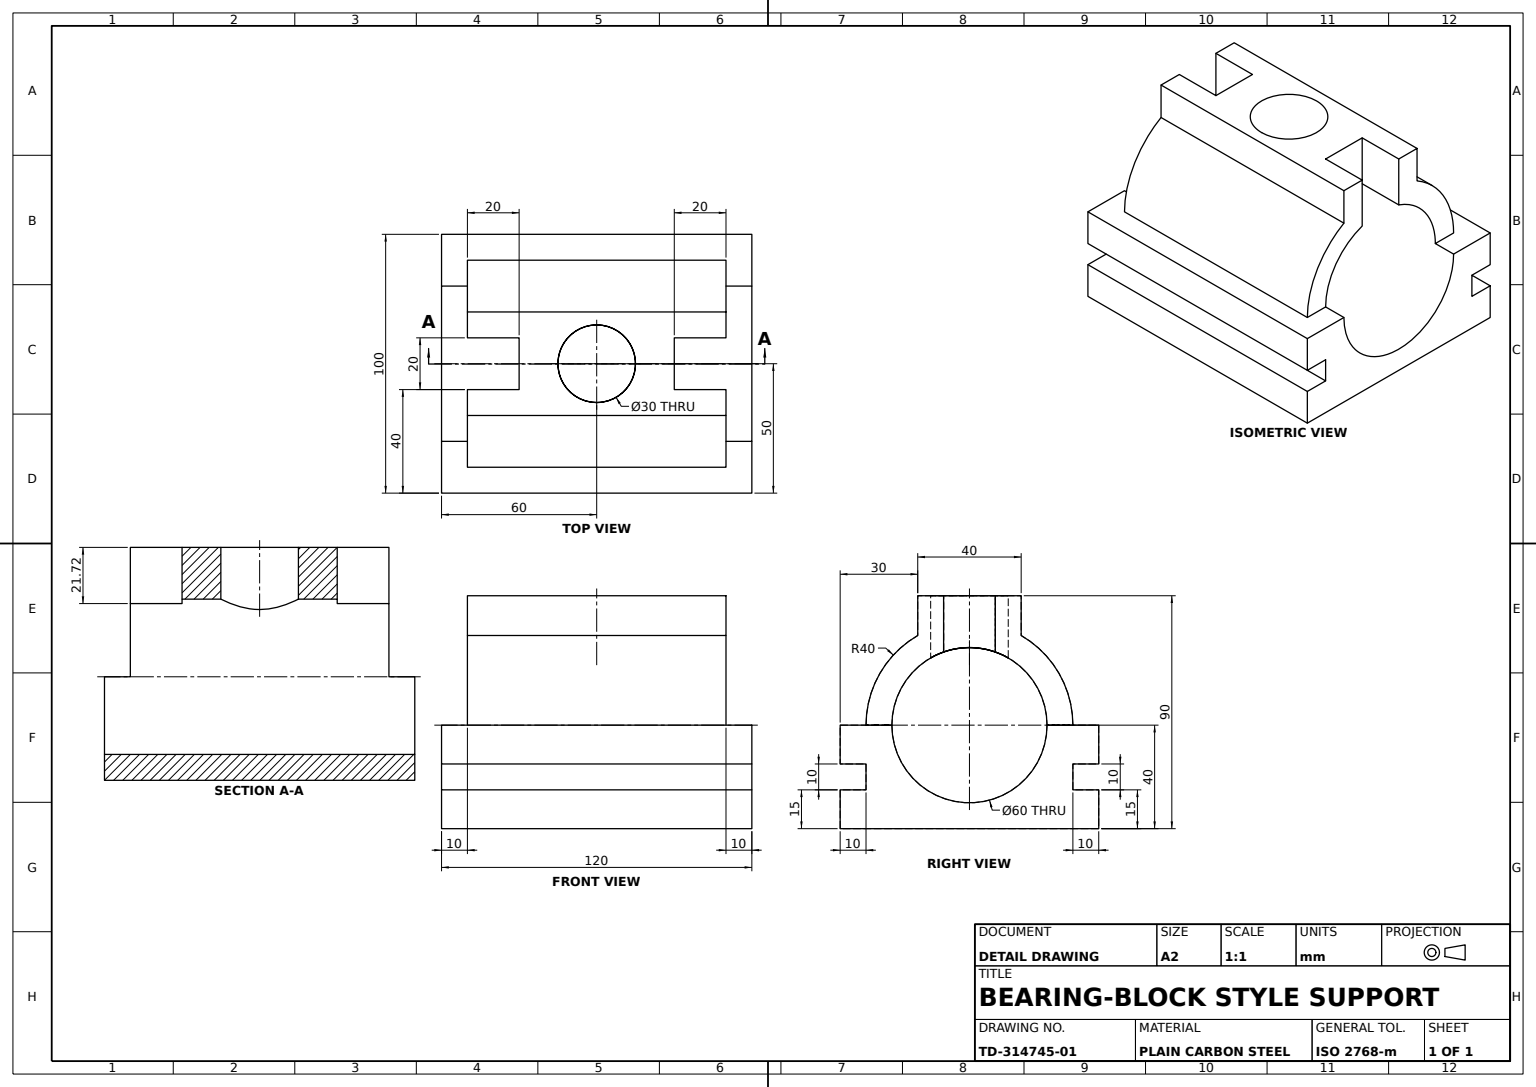
ISO-10303-21;
HEADER;
FILE_DESCRIPTION((''),'2;1');
FILE_NAME('','',(''),(''),'','','');
FILE_SCHEMA(('AUTOMOTIVE_DESIGN'));
ENDSEC;
DATA;
#1=APPLICATION_CONTEXT('');
#2=PRODUCT_CONTEXT('',#1,'mechanical');
#3=PRODUCT('','','',(#2));
#4=PRODUCT_DEFINITION_FORMATION('','',#3);
#5=PRODUCT_DEFINITION_CONTEXT('',#1,'design');
#6=PRODUCT_DEFINITION('','',#4,#5);
#7=PRODUCT_DEFINITION_SHAPE('','',#6);
#8=(LENGTH_UNIT()NAMED_UNIT(*)SI_UNIT(.MILLI.,.METRE.));
#9=(NAMED_UNIT(*)PLANE_ANGLE_UNIT()SI_UNIT($,.RADIAN.));
#10=(NAMED_UNIT(*)SI_UNIT($,.STERADIAN.)SOLID_ANGLE_UNIT());
#11=UNCERTAINTY_MEASURE_WITH_UNIT(LENGTH_MEASURE(1.E-05),#8,'distance_accuracy_value','');
#12=(GEOMETRIC_REPRESENTATION_CONTEXT(3)GLOBAL_UNCERTAINTY_ASSIGNED_CONTEXT((#11))GLOBAL_UNIT_ASSIGNED_CONTEXT((#8,#9,#10))REPRESENTATION_CONTEXT('',''));
#13=CARTESIAN_POINT('',(65.,65.980762,-60.));
#14=VERTEX_POINT('',#13);
#15=CARTESIAN_POINT('',(35.,65.980762,-60.));
#16=VERTEX_POINT('',#15);
#17=CARTESIAN_POINT('',(65.,65.980762,-59.503514));
#18=CARTESIAN_POINT('',(64.975416,65.995004,-59.005113));
#19=CARTESIAN_POINT('',(64.875156,66.052506,-58.004351));
#20=CARTESIAN_POINT('',(64.800107,66.095393,-57.509543));
#21=CARTESIAN_POINT('',(64.505151,66.261216,-56.052494));
#22=CARTESIAN_POINT('',(64.215664,66.421584,-55.11219));
#23=CARTESIAN_POINT('',(63.451904,66.818491,-53.290153));
#24=CARTESIAN_POINT('',(62.989124,67.048728,-52.435825));
#25=CARTESIAN_POINT('',(62.180532,67.417556,-51.232551));
#26=CARTESIAN_POINT('',(61.891675,67.544511,-50.844443));
#27=CARTESIAN_POINT('',(61.274128,67.802987,-50.093931));
#28=CARTESIAN_POINT('',(60.947936,67.933407,-49.734782));
#29=CARTESIAN_POINT('',(59.926264,68.319595,-48.712961));
#30=CARTESIAN_POINT('',(59.184727,68.571758,-48.101049));
#31=CARTESIAN_POINT('',(57.975732,68.923413,-47.286867));
#32=CARTESIAN_POINT('',(57.553955,69.036776,-47.03168));
#33=CARTESIAN_POINT('',(56.69248,69.247347,-46.566822));
#34=CARTESIAN_POINT('',(56.252173,69.344857,-46.356378));
#35=CARTESIAN_POINT('',(54.902311,69.610955,-45.790156));
#36=CARTESIAN_POINT('',(53.964123,69.753262,-45.498737));
#37=CARTESIAN_POINT('',(52.49344,69.900259,-45.200237));
#38=CARTESIAN_POINT('',(51.995929,69.937639,-45.125052));
#39=CARTESIAN_POINT('',(51.005292,69.987253,-45.025448));
#40=CARTESIAN_POINT('',(50.50939,69.999784,-45.000433));
#41=CARTESIAN_POINT('',(49.516426,70.000211,-44.999578));
#42=CARTESIAN_POINT('',(49.019365,69.988108,-45.023737));
#43=CARTESIAN_POINT('',(48.024058,69.939003,-45.122307));
#44=CARTESIAN_POINT('',(47.524118,69.901685,-45.197361));
#45=CARTESIAN_POINT('',(46.059254,69.756237,-45.492658));
#46=CARTESIAN_POINT('',(45.117292,69.614488,-45.78273));
#47=CARTESIAN_POINT('',(43.753408,69.34612,-46.353645));
#48=CARTESIAN_POINT('',(43.30559,69.246907,-46.56778));
#49=CARTESIAN_POINT('',(42.444004,69.036246,-47.032865));
#50=CARTESIAN_POINT('',(42.028081,68.924446,-47.284536));
#51=CARTESIAN_POINT('',(41.224502,68.690865,-47.825224));
#52=CARTESIAN_POINT('',(40.836849,68.569076,-48.114244));
#53=CARTESIAN_POINT('',(40.089257,68.318415,-48.730053));
#54=CARTESIAN_POINT('',(39.727696,68.188892,-49.058595));
#55=CARTESIAN_POINT('',(38.701032,67.800518,-50.086794));
#56=CARTESIAN_POINT('',(38.091001,67.541355,-50.82898));
#57=CARTESIAN_POINT('',(37.283022,67.172892,-52.030594));
#58=CARTESIAN_POINT('',(37.031694,67.053469,-52.445978));
#59=CARTESIAN_POINT('',(36.566237,66.825383,-53.308645));
#60=CARTESIAN_POINT('',(36.354634,66.717956,-53.751628));
#61=CARTESIAN_POINT('',(35.788686,66.423841,-55.101913));
#62=CARTESIAN_POINT('',(35.499327,66.2637,-56.036017));
#63=CARTESIAN_POINT('',(35.202669,66.09697,-57.493076));
#64=CARTESIAN_POINT('',(35.126663,66.053546,-57.990752));
#65=CARTESIAN_POINT('',(35.025442,65.9955,-58.9921));
#66=CARTESIAN_POINT('',(35.,65.980762,-59.495938));
#67=B_SPLINE_CURVE_WITH_KNOTS('',3,(#13,#17,#18,#19,#20,#21,#22,#23,#24,#25,#26,#27,#28,#29,#30,#31,#32,#33,#34,#35,#36,#37,#38,#39,#40,#41,#42,#43,#44,#45,#46,#47,#48,#49,#50,#51,#52,#53,#54,#55,#56,#57,#58,#59,#60,#61,#62,#63,#64,#65,#66,#15),.UNSPECIFIED.,.F.,.F.,(4,2,2,2,2,2,2,2,2,2,2,2,2,2,2,2,2,2,2,2,2,2,2,2,2,4),(0.047708954,0.049197223,0.050685492,0.053662031,0.05663857,0.058126839,0.059615109,0.062591647,0.064079917,0.065568186,0.068544725,0.070032994,0.071521263,0.073009533,0.074497802,0.077474341,0.07896261,0.08045088,0.081939149,0.083427418,0.086403957,0.087892226,0.089380496,0.092357035,0.093845304,0.095333573),.UNSPECIFIED.);
#68=EDGE_CURVE('',#14,#16,#67,.T.);
#69=ORIENTED_EDGE('',*,*,#68,.F.);
#70=CARTESIAN_POINT('',(35.,65.980762,-61.00991));
#71=CARTESIAN_POINT('',(35.100904,66.039726,-61.998787));
#72=CARTESIAN_POINT('',(35.394482,66.204798,-63.453028));
#73=CARTESIAN_POINT('',(35.516241,66.272578,-63.932899));
#74=CARTESIAN_POINT('',(35.808323,66.431496,-64.88296));
#75=CARTESIAN_POINT('',(35.977469,66.521955,-65.348671));
#76=CARTESIAN_POINT('',(36.545369,66.817065,-66.703103));
#77=CARTESIAN_POINT('',(37.006104,67.046531,-67.556891));
#78=CARTESIAN_POINT('',(37.820536,67.418054,-68.76913));
#79=CARTESIAN_POINT('',(38.11221,67.546163,-69.160437));
#80=CARTESIAN_POINT('',(38.725978,67.803005,-69.906038));
#81=CARTESIAN_POINT('',(39.049317,67.932321,-70.262249));
#82=CARTESIAN_POINT('',(39.729091,68.189368,-70.942561));
#83=CARTESIAN_POINT('',(40.085524,68.317106,-71.266661));
#84=CARTESIAN_POINT('',(40.832809,68.567778,-71.882638));
#85=CARTESIAN_POINT('',(41.225935,68.691341,-72.175924));
#86=CARTESIAN_POINT('',(42.438815,69.043717,-72.991454));
#87=CARTESIAN_POINT('',(43.292713,69.255022,-73.45243));
#88=CARTESIAN_POINT('',(44.644725,69.521721,-74.019983));
#89=CARTESIAN_POINT('',(45.107337,69.602244,-74.18835));
#90=CARTESIAN_POINT('',(46.058083,69.743777,-74.481324));
#91=CARTESIAN_POINT('',(46.544404,69.804329,-74.604976));
#92=CARTESIAN_POINT('',(48.004312,69.949522,-74.899769));
#93=CARTESIAN_POINT('',(48.990566,69.999671,-74.999343));
#94=CARTESIAN_POINT('',(50.489993,70.000162,-75.000324));
#95=CARTESIAN_POINT('',(50.996371,69.987604,-74.975255));
#96=CARTESIAN_POINT('',(51.993415,69.93786,-74.875393));
#97=CARTESIAN_POINT('',(52.485426,69.900852,-74.800954));
#98=CARTESIAN_POINT('',(53.456927,69.80416,-74.604631));
#99=CARTESIAN_POINT('',(53.936417,69.744472,-74.482743));
#100=CARTESIAN_POINT('',(54.883034,69.6038,-74.191589));
#101=CARTESIAN_POINT('',(55.352688,69.522267,-74.021153));
#102=CARTESIAN_POINT('',(56.719013,69.252639,-73.447338));
#103=CARTESIAN_POINT('',(57.575449,69.039935,-72.982988));
#104=CARTESIAN_POINT('',(58.784985,68.687983,-72.168007));
#105=CARTESIAN_POINT('',(59.177289,68.564556,-71.874929));
#106=CARTESIAN_POINT('',(59.927306,68.312631,-71.25545));
#107=CARTESIAN_POINT('',(60.284308,68.184483,-70.929994));
#108=CARTESIAN_POINT('',(61.303858,67.7984,-69.90706));
#109=CARTESIAN_POINT('',(61.915532,67.538642,-69.163617));
#110=CARTESIAN_POINT('',(62.730469,67.166603,-67.948151));
#111=CARTESIAN_POINT('',(62.982388,67.046685,-67.529497));
#112=CARTESIAN_POINT('',(63.442131,66.821161,-66.674193));
#113=CARTESIAN_POINT('',(63.650903,66.715119,-66.236145));
#114=CARTESIAN_POINT('',(64.026289,66.519954,-65.338527));
#115=CARTESIAN_POINT('',(64.192907,66.430826,-64.878958));
#116=CARTESIAN_POINT('',(64.41013,66.312639,-64.172394));
#117=CARTESIAN_POINT('',(64.477074,66.27583,-63.933999));
#118=CARTESIAN_POINT('',(64.599699,66.207894,-63.451206));
#119=CARTESIAN_POINT('',(64.655474,66.176713,-63.206163));
#120=CARTESIAN_POINT('',(64.902037,66.038059,-61.981814));
#121=CARTESIAN_POINT('',(65.,65.980762,-60.994731));
#122=B_SPLINE_CURVE_WITH_KNOTS('',3,(#15,#70,#71,#72,#73,#74,#75,#76,#77,#78,#79,#80,#81,#82,#83,#84,#85,#86,#87,#88,#89,#90,#91,#92,#93,#94,#95,#96,#97,#98,#99,#100,#101,#102,#103,#104,#105,#106,#107,#108,#109,#110,#111,#112,#113,#114,#115,#116,#117,#118,#119,#120,#121,#13),.UNSPECIFIED.,.F.,.F.,(4,2,2,2,2,2,2,2,2,2,2,2,2,2,2,2,2,2,2,2,2,2,2,2,2,2,4),(0.,0.00298181,0.004472714,0.005963619,0.008945429,0.010436334,0.011927238,0.013418143,0.014909048,0.017890858,0.019381762,0.020872667,0.023854477,0.025345382,0.026836286,0.028327191,0.029818096,0.032799906,0.03429081,0.035781715,0.038763525,0.04025443,0.041745334,0.043236239,0.043981692,0.044727144,0.047708954),.UNSPECIFIED.);
#123=EDGE_CURVE('',#16,#14,#122,.T.);
#124=ORIENTED_EDGE('',*,*,#123,.F.);
#125=EDGE_LOOP('',(#69,#124));
#126=FACE_BOUND('',#125,.T.);
#127=CARTESIAN_POINT('',(40.,68.284271,-10.));
#128=VERTEX_POINT('',#127);
#129=CARTESIAN_POINT('',(40.,68.284271,-30.));
#130=VERTEX_POINT('',#129);
#131=CARTESIAN_POINT('',(40.,68.284271,-120.));
#132=DIRECTION('',(0.,0.,-1.));
#133=VECTOR('',#132,1000.);
#134=LINE('',#131,#133);
#135=EDGE_CURVE('',#128,#130,#134,.T.);
#136=ORIENTED_EDGE('',*,*,#135,.F.);
#137=CARTESIAN_POINT('',(20.,40.,-10.));
#138=VERTEX_POINT('',#137);
#139=CARTESIAN_POINT('',(50.,40.,-10.));
#140=DIRECTION('',(0.,0.,1.));
#141=DIRECTION('',(1.,0.,0.));
#142=AXIS2_PLACEMENT_3D('',#139,#140,#141);
#143=CIRCLE('',#142,30.);
#144=EDGE_CURVE('',#128,#138,#143,.T.);
#145=ORIENTED_EDGE('',*,*,#144,.T.);
#146=CARTESIAN_POINT('',(20.,40.,-110.));
#147=VERTEX_POINT('',#146);
#148=CARTESIAN_POINT('',(20.,40.,-120.));
#149=VECTOR('',#140,1000.);
#150=LINE('',#148,#149);
#151=EDGE_CURVE('',#147,#138,#150,.T.);
#152=ORIENTED_EDGE('',*,*,#151,.F.);
#153=CARTESIAN_POINT('',(40.,68.284271,-110.));
#154=VERTEX_POINT('',#153);
#155=CARTESIAN_POINT('',(50.,40.,-110.));
#156=AXIS2_PLACEMENT_3D('',#155,#140,#141);
#157=CIRCLE('',#156,30.);
#158=EDGE_CURVE('',#154,#147,#157,.T.);
#159=ORIENTED_EDGE('',*,*,#158,.F.);
#160=CARTESIAN_POINT('',(40.,68.284271,-90.));
#161=VERTEX_POINT('',#160);
#162=EDGE_CURVE('',#161,#154,#134,.T.);
#163=ORIENTED_EDGE('',*,*,#162,.F.);
#164=CARTESIAN_POINT('',(60.,68.284271,-90.));
#165=VERTEX_POINT('',#164);
#166=CARTESIAN_POINT('',(50.,40.,-90.));
#167=AXIS2_PLACEMENT_3D('',#166,#140,#141);
#168=CIRCLE('',#167,30.);
#169=EDGE_CURVE('',#165,#161,#168,.T.);
#170=ORIENTED_EDGE('',*,*,#169,.F.);
#171=CARTESIAN_POINT('',(60.,68.284271,-110.));
#172=VERTEX_POINT('',#171);
#173=CARTESIAN_POINT('',(60.,68.284271,-120.));
#174=LINE('',#173,#149);
#175=EDGE_CURVE('',#172,#165,#174,.T.);
#176=ORIENTED_EDGE('',*,*,#175,.F.);
#177=CARTESIAN_POINT('',(80.,40.,-110.));
#178=VERTEX_POINT('',#177);
#179=EDGE_CURVE('',#178,#172,#157,.T.);
#180=ORIENTED_EDGE('',*,*,#179,.F.);
#181=CARTESIAN_POINT('',(80.,40.,-10.));
#182=VERTEX_POINT('',#181);
#183=CARTESIAN_POINT('',(80.,40.,-120.));
#184=LINE('',#183,#149);
#185=EDGE_CURVE('',#178,#182,#184,.T.);
#186=ORIENTED_EDGE('',*,*,#185,.T.);
#187=CARTESIAN_POINT('',(60.,68.284271,-10.));
#188=VERTEX_POINT('',#187);
#189=EDGE_CURVE('',#182,#188,#143,.T.);
#190=ORIENTED_EDGE('',*,*,#189,.T.);
#191=CARTESIAN_POINT('',(60.,68.284271,-30.));
#192=VERTEX_POINT('',#191);
#193=EDGE_CURVE('',#192,#188,#174,.T.);
#194=ORIENTED_EDGE('',*,*,#193,.F.);
#195=CARTESIAN_POINT('',(50.,40.,-30.));
#196=DIRECTION('',(-1.,0.,0.));
#197=AXIS2_PLACEMENT_3D('',#195,#132,#196);
#198=CIRCLE('',#197,30.);
#199=EDGE_CURVE('',#130,#192,#198,.T.);
#200=ORIENTED_EDGE('',*,*,#199,.F.);
#201=EDGE_LOOP('',(#136,#145,#152,#159,#163,#170,#176,#180,#186,#190,#194,#200));
#202=FACE_OUTER_BOUND('',#201,.T.);
#203=CARTESIAN_POINT('',(50.,40.,-120.));
#204=AXIS2_PLACEMENT_3D('',#203,#140,#141);
#205=CYLINDRICAL_SURFACE('',#204,30.);
#206=ADVANCED_FACE('',(#126,#202),#205,.F.);
#207=CARTESIAN_POINT('',(80.,40.,0.));
#208=VERTEX_POINT('',#207);
#209=EDGE_CURVE('',#182,#208,#184,.T.);
#210=ORIENTED_EDGE('',*,*,#209,.T.);
#211=CARTESIAN_POINT('',(100.,40.,0.));
#212=VERTEX_POINT('',#211);
#213=VECTOR('',#196,1000.);
#214=LINE('',#211,#213);
#215=EDGE_CURVE('',#212,#208,#214,.T.);
#216=ORIENTED_EDGE('',*,*,#215,.F.);
#217=CARTESIAN_POINT('',(100.,40.,-120.));
#218=VERTEX_POINT('',#217);
#219=LINE('',#217,#149);
#220=EDGE_CURVE('',#218,#212,#219,.T.);
#221=ORIENTED_EDGE('',*,*,#220,.F.);
#222=VERTEX_POINT('',#183);
#223=LINE('',#217,#213);
#224=EDGE_CURVE('',#218,#222,#223,.T.);
#225=ORIENTED_EDGE('',*,*,#224,.T.);
#226=EDGE_CURVE('',#222,#178,#184,.T.);
#227=ORIENTED_EDGE('',*,*,#226,.T.);
#228=CARTESIAN_POINT('',(90.,40.,-110.));
#229=VERTEX_POINT('',#228);
#230=CARTESIAN_POINT('',(0.,40.,-110.));
#231=VECTOR('',#141,1000.);
#232=LINE('',#230,#231);
#233=EDGE_CURVE('',#178,#229,#232,.T.);
#234=ORIENTED_EDGE('',*,*,#233,.T.);
#235=CARTESIAN_POINT('',(90.,40.,-10.));
#236=VERTEX_POINT('',#235);
#237=LINE('',#228,#149);
#238=EDGE_CURVE('',#229,#236,#237,.T.);
#239=ORIENTED_EDGE('',*,*,#238,.T.);
#240=CARTESIAN_POINT('',(0.,40.,-10.));
#241=LINE('',#240,#231);
#242=EDGE_CURVE('',#182,#236,#241,.T.);
#243=ORIENTED_EDGE('',*,*,#242,.F.);
#244=EDGE_LOOP('',(#210,#216,#221,#225,#227,#234,#239,#243));
#245=FACE_OUTER_BOUND('',#244,.T.);
#246=DIRECTION('',(0.,1.,0.));
#247=AXIS2_PLACEMENT_3D('',#217,#246,#140);
#248=PLANE('',#247);
#249=ADVANCED_FACE('',(#245),#248,.T.);
#250=CARTESIAN_POINT('',(60.,90.,-10.));
#251=VERTEX_POINT('',#250);
#252=CARTESIAN_POINT('',(70.,90.,-10.));
#253=VERTEX_POINT('',#252);
#254=CARTESIAN_POINT('',(0.,90.,-10.));
#255=LINE('',#254,#231);
#256=EDGE_CURVE('',#251,#253,#255,.T.);
#257=ORIENTED_EDGE('',*,*,#256,.T.);
#258=CARTESIAN_POINT('',(70.,90.,-110.));
#259=VERTEX_POINT('',#258);
#260=LINE('',#258,#149);
#261=EDGE_CURVE('',#259,#253,#260,.T.);
#262=ORIENTED_EDGE('',*,*,#261,.F.);
#263=CARTESIAN_POINT('',(60.,90.,-110.));
#264=VERTEX_POINT('',#263);
#265=CARTESIAN_POINT('',(0.,90.,-110.));
#266=LINE('',#265,#231);
#267=EDGE_CURVE('',#264,#259,#266,.T.);
#268=ORIENTED_EDGE('',*,*,#267,.F.);
#269=CARTESIAN_POINT('',(60.,90.,-90.));
#270=VERTEX_POINT('',#269);
#271=LINE('',#263,#133);
#272=EDGE_CURVE('',#270,#264,#271,.T.);
#273=ORIENTED_EDGE('',*,*,#272,.F.);
#274=CARTESIAN_POINT('',(40.,90.,-90.));
#275=VERTEX_POINT('',#274);
#276=LINE('',#274,#231);
#277=EDGE_CURVE('',#275,#270,#276,.T.);
#278=ORIENTED_EDGE('',*,*,#277,.F.);
#279=CARTESIAN_POINT('',(40.,90.,-110.));
#280=VERTEX_POINT('',#279);
#281=LINE('',#279,#149);
#282=EDGE_CURVE('',#280,#275,#281,.T.);
#283=ORIENTED_EDGE('',*,*,#282,.F.);
#284=CARTESIAN_POINT('',(30.,90.,-110.));
#285=VERTEX_POINT('',#284);
#286=EDGE_CURVE('',#285,#280,#266,.T.);
#287=ORIENTED_EDGE('',*,*,#286,.F.);
#288=CARTESIAN_POINT('',(30.,90.,-10.));
#289=VERTEX_POINT('',#288);
#290=LINE('',#284,#149);
#291=EDGE_CURVE('',#285,#289,#290,.T.);
#292=ORIENTED_EDGE('',*,*,#291,.T.);
#293=CARTESIAN_POINT('',(40.,90.,-10.));
#294=VERTEX_POINT('',#293);
#295=EDGE_CURVE('',#289,#294,#255,.T.);
#296=ORIENTED_EDGE('',*,*,#295,.T.);
#297=CARTESIAN_POINT('',(40.,90.,-30.));
#298=VERTEX_POINT('',#297);
#299=LINE('',#293,#149);
#300=EDGE_CURVE('',#298,#294,#299,.T.);
#301=ORIENTED_EDGE('',*,*,#300,.F.);
#302=CARTESIAN_POINT('',(60.,90.,-30.));
#303=VERTEX_POINT('',#302);
#304=LINE('',#297,#213);
#305=EDGE_CURVE('',#303,#298,#304,.T.);
#306=ORIENTED_EDGE('',*,*,#305,.F.);
#307=LINE('',#250,#133);
#308=EDGE_CURVE('',#251,#303,#307,.T.);
#309=ORIENTED_EDGE('',*,*,#308,.F.);
#310=EDGE_LOOP('',(#257,#262,#268,#273,#278,#283,#287,#292,#296,#301,#306,#309));
#311=FACE_OUTER_BOUND('',#310,.T.);
#312=CARTESIAN_POINT('',(35.,90.,-60.));
#313=VERTEX_POINT('',#312);
#314=CARTESIAN_POINT('',(65.,90.,-60.));
#315=VERTEX_POINT('',#314);
#316=CARTESIAN_POINT('',(50.,90.,-60.));
#317=AXIS2_PLACEMENT_3D('',#316,#246,#196);
#318=CIRCLE('',#317,15.);
#319=EDGE_CURVE('',#313,#315,#318,.T.);
#320=ORIENTED_EDGE('',*,*,#319,.F.);
#321=EDGE_CURVE('',#315,#313,#318,.T.);
#322=ORIENTED_EDGE('',*,*,#321,.F.);
#323=EDGE_LOOP('',(#320,#322));
#324=FACE_BOUND('',#323,.T.);
#325=DIRECTION('',(0.,-1.,0.));
#326=AXIS2_PLACEMENT_3D('',#265,#325,#141);
#327=PLANE('',#326);
#328=ADVANCED_FACE('',(#311,#324),#327,.F.);
#329=ORIENTED_EDGE('',*,*,#135,.T.);
#330=CARTESIAN_POINT('',(40.,60.,-30.));
#331=VECTOR('',#246,1000.);
#332=LINE('',#330,#331);
#333=EDGE_CURVE('',#130,#298,#332,.T.);
#334=ORIENTED_EDGE('',*,*,#333,.T.);
#335=ORIENTED_EDGE('',*,*,#300,.T.);
#336=CARTESIAN_POINT('',(40.,0.,-10.));
#337=VECTOR('',#325,1000.);
#338=LINE('',#336,#337);
#339=EDGE_CURVE('',#294,#128,#338,.T.);
#340=ORIENTED_EDGE('',*,*,#339,.T.);
#341=EDGE_LOOP('',(#329,#334,#335,#340));
#342=FACE_OUTER_BOUND('',#341,.T.);
#343=CARTESIAN_POINT('',(40.,60.,-10.));
#344=AXIS2_PLACEMENT_3D('',#343,#196,#325);
#345=PLANE('',#344);
#346=ADVANCED_FACE('',(#342),#345,.F.);
#347=CARTESIAN_POINT('',(10.,15.,-120.));
#348=VERTEX_POINT('',#347);
#349=CARTESIAN_POINT('',(10.,15.,0.));
#350=VERTEX_POINT('',#349);
#351=LINE('',#347,#149);
#352=EDGE_CURVE('',#348,#350,#351,.T.);
#353=ORIENTED_EDGE('',*,*,#352,.F.);
#354=CARTESIAN_POINT('',(0.,15.,-120.));
#355=VERTEX_POINT('',#354);
#356=LINE('',#347,#213);
#357=EDGE_CURVE('',#348,#355,#356,.T.);
#358=ORIENTED_EDGE('',*,*,#357,.T.);
#359=CARTESIAN_POINT('',(0.,15.,0.));
#360=VERTEX_POINT('',#359);
#361=LINE('',#354,#149);
#362=EDGE_CURVE('',#355,#360,#361,.T.);
#363=ORIENTED_EDGE('',*,*,#362,.T.);
#364=LINE('',#349,#213);
#365=EDGE_CURVE('',#350,#360,#364,.T.);
#366=ORIENTED_EDGE('',*,*,#365,.F.);
#367=EDGE_LOOP('',(#353,#358,#363,#366));
#368=FACE_OUTER_BOUND('',#367,.T.);
#369=AXIS2_PLACEMENT_3D('',#347,#246,#140);
#370=PLANE('',#369);
#371=ADVANCED_FACE('',(#368),#370,.T.);
#372=VERTEX_POINT('',#148);
#373=AXIS2_PLACEMENT_3D('',#203,#132,#141);
#374=CIRCLE('',#373,30.);
#375=EDGE_CURVE('',#222,#372,#374,.T.);
#376=ORIENTED_EDGE('',*,*,#375,.T.);
#377=EDGE_CURVE('',#372,#147,#150,.T.);
#378=ORIENTED_EDGE('',*,*,#377,.T.);
#379=ORIENTED_EDGE('',*,*,#151,.T.);
#380=CARTESIAN_POINT('',(20.,40.,0.));
#381=VERTEX_POINT('',#380);
#382=EDGE_CURVE('',#138,#381,#150,.T.);
#383=ORIENTED_EDGE('',*,*,#382,.T.);
#384=CARTESIAN_POINT('',(50.,40.,0.));
#385=AXIS2_PLACEMENT_3D('',#384,#132,#141);
#386=CIRCLE('',#385,30.);
#387=EDGE_CURVE('',#208,#381,#386,.T.);
#388=ORIENTED_EDGE('',*,*,#387,.F.);
#389=ORIENTED_EDGE('',*,*,#209,.F.);
#390=ORIENTED_EDGE('',*,*,#185,.F.);
#391=ORIENTED_EDGE('',*,*,#226,.F.);
#392=EDGE_LOOP('',(#376,#378,#379,#383,#388,#389,#390,#391));
#393=FACE_OUTER_BOUND('',#392,.T.);
#394=ADVANCED_FACE('',(#393),#205,.F.);
#395=ORIENTED_EDGE('',*,*,#339,.F.);
#396=ORIENTED_EDGE('',*,*,#295,.F.);
#397=CARTESIAN_POINT('',(30.,74.641016,-10.));
#398=VERTEX_POINT('',#397);
#399=CARTESIAN_POINT('',(30.,0.,-10.));
#400=LINE('',#399,#337);
#401=EDGE_CURVE('',#289,#398,#400,.T.);
#402=ORIENTED_EDGE('',*,*,#401,.T.);
#403=CARTESIAN_POINT('',(10.,40.,-10.));
#404=VERTEX_POINT('',#403);
#405=CIRCLE('',#142,40.);
#406=EDGE_CURVE('',#398,#404,#405,.T.);
#407=ORIENTED_EDGE('',*,*,#406,.T.);
#408=EDGE_CURVE('',#404,#138,#241,.T.);
#409=ORIENTED_EDGE('',*,*,#408,.T.);
#410=ORIENTED_EDGE('',*,*,#144,.F.);
#411=EDGE_LOOP('',(#395,#396,#402,#407,#409,#410));
#412=FACE_OUTER_BOUND('',#411,.T.);
#413=CARTESIAN_POINT('',(0.,0.,-10.));
#414=AXIS2_PLACEMENT_3D('',#413,#140,#141);
#415=PLANE('',#414);
#416=ADVANCED_FACE('',(#412),#415,.T.);
#417=CARTESIAN_POINT('',(100.,25.,0.));
#418=VERTEX_POINT('',#417);
#419=LINE('',#417,#331);
#420=EDGE_CURVE('',#418,#212,#419,.T.);
#421=ORIENTED_EDGE('',*,*,#420,.F.);
#422=CARTESIAN_POINT('',(100.,25.,-120.));
#423=VERTEX_POINT('',#422);
#424=LINE('',#422,#149);
#425=EDGE_CURVE('',#423,#418,#424,.T.);
#426=ORIENTED_EDGE('',*,*,#425,.F.);
#427=LINE('',#422,#331);
#428=EDGE_CURVE('',#423,#218,#427,.T.);
#429=ORIENTED_EDGE('',*,*,#428,.T.);
#430=ORIENTED_EDGE('',*,*,#220,.T.);
#431=EDGE_LOOP('',(#421,#426,#429,#430));
#432=FACE_OUTER_BOUND('',#431,.T.);
#433=AXIS2_PLACEMENT_3D('',#422,#141,#132);
#434=PLANE('',#433);
#435=ADVANCED_FACE('',(#432),#434,.T.);
#436=ORIENTED_EDGE('',*,*,#401,.F.);
#437=ORIENTED_EDGE('',*,*,#291,.F.);
#438=CARTESIAN_POINT('',(30.,74.641016,-110.));
#439=VERTEX_POINT('',#438);
#440=CARTESIAN_POINT('',(30.,0.,-110.));
#441=LINE('',#440,#337);
#442=EDGE_CURVE('',#285,#439,#441,.T.);
#443=ORIENTED_EDGE('',*,*,#442,.T.);
#444=LINE('',#438,#149);
#445=EDGE_CURVE('',#439,#398,#444,.T.);
#446=ORIENTED_EDGE('',*,*,#445,.T.);
#447=EDGE_LOOP('',(#436,#437,#443,#446));
#448=FACE_OUTER_BOUND('',#447,.T.);
#449=AXIS2_PLACEMENT_3D('',#440,#196,#325);
#450=PLANE('',#449);
#451=ADVANCED_FACE('',(#448),#450,.T.);
#452=CARTESIAN_POINT('',(100.,15.,-120.));
#453=VERTEX_POINT('',#452);
#454=CARTESIAN_POINT('',(90.,15.,-120.));
#455=VERTEX_POINT('',#454);
#456=LINE('',#452,#213);
#457=EDGE_CURVE('',#453,#455,#456,.T.);
#458=ORIENTED_EDGE('',*,*,#457,.T.);
#459=CARTESIAN_POINT('',(90.,15.,0.));
#460=VERTEX_POINT('',#459);
#461=LINE('',#454,#149);
#462=EDGE_CURVE('',#455,#460,#461,.T.);
#463=ORIENTED_EDGE('',*,*,#462,.T.);
#464=CARTESIAN_POINT('',(100.,15.,0.));
#465=VERTEX_POINT('',#464);
#466=LINE('',#464,#213);
#467=EDGE_CURVE('',#465,#460,#466,.T.);
#468=ORIENTED_EDGE('',*,*,#467,.F.);
#469=LINE('',#452,#149);
#470=EDGE_CURVE('',#453,#465,#469,.T.);
#471=ORIENTED_EDGE('',*,*,#470,.F.);
#472=EDGE_LOOP('',(#458,#463,#468,#471));
#473=FACE_OUTER_BOUND('',#472,.T.);
#474=AXIS2_PLACEMENT_3D('',#452,#246,#140);
#475=PLANE('',#474);
#476=ADVANCED_FACE('',(#473),#475,.T.);
#477=CARTESIAN_POINT('',(0.,40.,0.));
#478=VERTEX_POINT('',#477);
#479=LINE('',#380,#213);
#480=EDGE_CURVE('',#381,#478,#479,.T.);
#481=ORIENTED_EDGE('',*,*,#480,.F.);
#482=ORIENTED_EDGE('',*,*,#382,.F.);
#483=ORIENTED_EDGE('',*,*,#408,.F.);
#484=CARTESIAN_POINT('',(10.,40.,-110.));
#485=VERTEX_POINT('',#484);
#486=LINE('',#484,#149);
#487=EDGE_CURVE('',#485,#404,#486,.T.);
#488=ORIENTED_EDGE('',*,*,#487,.F.);
#489=EDGE_CURVE('',#485,#147,#232,.T.);
#490=ORIENTED_EDGE('',*,*,#489,.T.);
#491=ORIENTED_EDGE('',*,*,#377,.F.);
#492=CARTESIAN_POINT('',(0.,40.,-120.));
#493=VERTEX_POINT('',#492);
#494=LINE('',#148,#213);
#495=EDGE_CURVE('',#372,#493,#494,.T.);
#496=ORIENTED_EDGE('',*,*,#495,.T.);
#497=LINE('',#492,#149);
#498=EDGE_CURVE('',#493,#478,#497,.T.);
#499=ORIENTED_EDGE('',*,*,#498,.T.);
#500=EDGE_LOOP('',(#481,#482,#483,#488,#490,#491,#496,#499));
#501=FACE_OUTER_BOUND('',#500,.T.);
#502=AXIS2_PLACEMENT_3D('',#148,#246,#140);
#503=PLANE('',#502);
#504=ADVANCED_FACE('',(#501),#503,.T.);
#505=ORIENTED_EDGE('',*,*,#352,.T.);
#506=CARTESIAN_POINT('',(10.,25.,0.));
#507=VERTEX_POINT('',#506);
#508=LINE('',#506,#337);
#509=EDGE_CURVE('',#507,#350,#508,.T.);
#510=ORIENTED_EDGE('',*,*,#509,.F.);
#511=CARTESIAN_POINT('',(10.,25.,-120.));
#512=VERTEX_POINT('',#511);
#513=LINE('',#511,#149);
#514=EDGE_CURVE('',#512,#507,#513,.T.);
#515=ORIENTED_EDGE('',*,*,#514,.F.);
#516=LINE('',#511,#337);
#517=EDGE_CURVE('',#512,#348,#516,.T.);
#518=ORIENTED_EDGE('',*,*,#517,.T.);
#519=EDGE_LOOP('',(#505,#510,#515,#518));
#520=FACE_OUTER_BOUND('',#519,.T.);
#521=AXIS2_PLACEMENT_3D('',#511,#196,#140);
#522=PLANE('',#521);
#523=ADVANCED_FACE('',(#520),#522,.T.);
#524=CARTESIAN_POINT('',(35.,60.,-60.));
#525=LINE('',#524,#331);
#526=EDGE_CURVE('',#16,#313,#525,.T.);
#527=ORIENTED_EDGE('',*,*,#526,.F.);
#528=ORIENTED_EDGE('',*,*,#123,.T.);
#529=CARTESIAN_POINT('',(65.,60.,-60.));
#530=LINE('',#529,#331);
#531=EDGE_CURVE('',#14,#315,#530,.T.);
#532=ORIENTED_EDGE('',*,*,#531,.T.);
#533=ORIENTED_EDGE('',*,*,#321,.T.);
#534=EDGE_LOOP('',(#527,#528,#532,#533));
#535=FACE_OUTER_BOUND('',#534,.T.);
#536=CARTESIAN_POINT('',(50.,60.,-60.));
#537=AXIS2_PLACEMENT_3D('',#536,#246,#196);
#538=CYLINDRICAL_SURFACE('',#537,15.);
#539=ADVANCED_FACE('',(#535),#538,.F.);
#540=ORIENTED_EDGE('',*,*,#162,.T.);
#541=CARTESIAN_POINT('',(40.,0.,-110.));
#542=LINE('',#541,#337);
#543=EDGE_CURVE('',#280,#154,#542,.T.);
#544=ORIENTED_EDGE('',*,*,#543,.F.);
#545=ORIENTED_EDGE('',*,*,#282,.T.);
#546=CARTESIAN_POINT('',(40.,60.,-90.));
#547=LINE('',#546,#331);
#548=EDGE_CURVE('',#161,#275,#547,.T.);
#549=ORIENTED_EDGE('',*,*,#548,.F.);
#550=EDGE_LOOP('',(#540,#544,#545,#549));
#551=FACE_OUTER_BOUND('',#550,.T.);
#552=CARTESIAN_POINT('',(40.,60.,-110.));
#553=AXIS2_PLACEMENT_3D('',#552,#196,#325);
#554=PLANE('',#553);
#555=ADVANCED_FACE('',(#551),#554,.F.);
#556=ORIENTED_EDGE('',*,*,#526,.T.);
#557=ORIENTED_EDGE('',*,*,#319,.T.);
#558=ORIENTED_EDGE('',*,*,#531,.F.);
#559=ORIENTED_EDGE('',*,*,#68,.T.);
#560=EDGE_LOOP('',(#556,#557,#558,#559));
#561=FACE_OUTER_BOUND('',#560,.T.);
#562=ADVANCED_FACE('',(#561),#538,.F.);
#563=ORIENTED_EDGE('',*,*,#514,.T.);
#564=CARTESIAN_POINT('',(0.,25.,0.));
#565=VERTEX_POINT('',#564);
#566=LINE('',#564,#231);
#567=EDGE_CURVE('',#565,#507,#566,.T.);
#568=ORIENTED_EDGE('',*,*,#567,.F.);
#569=CARTESIAN_POINT('',(0.,25.,-120.));
#570=VERTEX_POINT('',#569);
#571=LINE('',#569,#149);
#572=EDGE_CURVE('',#570,#565,#571,.T.);
#573=ORIENTED_EDGE('',*,*,#572,.F.);
#574=LINE('',#569,#231);
#575=EDGE_CURVE('',#570,#512,#574,.T.);
#576=ORIENTED_EDGE('',*,*,#575,.T.);
#577=EDGE_LOOP('',(#563,#568,#573,#576));
#578=FACE_OUTER_BOUND('',#577,.T.);
#579=AXIS2_PLACEMENT_3D('',#569,#325,#132);
#580=PLANE('',#579);
#581=ADVANCED_FACE('',(#578),#580,.T.);
#582=CARTESIAN_POINT('',(0.,0.,-120.));
#583=VERTEX_POINT('',#582);
#584=CARTESIAN_POINT('',(100.,0.,-120.));
#585=VERTEX_POINT('',#584);
#586=LINE('',#582,#231);
#587=EDGE_CURVE('',#583,#585,#586,.T.);
#588=ORIENTED_EDGE('',*,*,#587,.F.);
#589=LINE('',#354,#337);
#590=EDGE_CURVE('',#355,#583,#589,.T.);
#591=ORIENTED_EDGE('',*,*,#590,.F.);
#592=ORIENTED_EDGE('',*,*,#357,.F.);
#593=ORIENTED_EDGE('',*,*,#517,.F.);
#594=ORIENTED_EDGE('',*,*,#575,.F.);
#595=LINE('',#492,#337);
#596=EDGE_CURVE('',#493,#570,#595,.T.);
#597=ORIENTED_EDGE('',*,*,#596,.F.);
#598=ORIENTED_EDGE('',*,*,#495,.F.);
#599=ORIENTED_EDGE('',*,*,#375,.F.);
#600=ORIENTED_EDGE('',*,*,#224,.F.);
#601=ORIENTED_EDGE('',*,*,#428,.F.);
#602=CARTESIAN_POINT('',(90.,25.,-120.));
#603=VERTEX_POINT('',#602);
#604=LINE('',#602,#231);
#605=EDGE_CURVE('',#603,#423,#604,.T.);
#606=ORIENTED_EDGE('',*,*,#605,.F.);
#607=LINE('',#454,#331);
#608=EDGE_CURVE('',#455,#603,#607,.T.);
#609=ORIENTED_EDGE('',*,*,#608,.F.);
#610=ORIENTED_EDGE('',*,*,#457,.F.);
#611=LINE('',#584,#331);
#612=EDGE_CURVE('',#585,#453,#611,.T.);
#613=ORIENTED_EDGE('',*,*,#612,.F.);
#614=EDGE_LOOP('',(#588,#591,#592,#593,#594,#597,#598,#599,#600,#601,#606,#609,#610,#613));
#615=FACE_OUTER_BOUND('',#614,.T.);
#616=PLANE('',#204);
#617=ADVANCED_FACE('',(#615),#616,.F.);
#618=CARTESIAN_POINT('',(70.,74.641016,-10.));
#619=VERTEX_POINT('',#618);
#620=EDGE_CURVE('',#236,#619,#405,.T.);
#621=ORIENTED_EDGE('',*,*,#620,.F.);
#622=ORIENTED_EDGE('',*,*,#238,.F.);
#623=CARTESIAN_POINT('',(70.,74.641016,-110.));
#624=VERTEX_POINT('',#623);
#625=CIRCLE('',#156,40.);
#626=EDGE_CURVE('',#229,#624,#625,.T.);
#627=ORIENTED_EDGE('',*,*,#626,.T.);
#628=LINE('',#623,#149);
#629=EDGE_CURVE('',#624,#619,#628,.T.);
#630=ORIENTED_EDGE('',*,*,#629,.T.);
#631=EDGE_LOOP('',(#621,#622,#627,#630));
#632=FACE_OUTER_BOUND('',#631,.T.);
#633=CYLINDRICAL_SURFACE('',#156,40.);
#634=ADVANCED_FACE('',(#632),#633,.T.);
#635=CARTESIAN_POINT('',(70.,0.,-110.));
#636=LINE('',#635,#337);
#637=EDGE_CURVE('',#259,#624,#636,.T.);
#638=ORIENTED_EDGE('',*,*,#637,.F.);
#639=ORIENTED_EDGE('',*,*,#261,.T.);
#640=CARTESIAN_POINT('',(70.,0.,-10.));
#641=LINE('',#640,#337);
#642=EDGE_CURVE('',#253,#619,#641,.T.);
#643=ORIENTED_EDGE('',*,*,#642,.T.);
#644=ORIENTED_EDGE('',*,*,#629,.F.);
#645=EDGE_LOOP('',(#638,#639,#643,#644));
#646=FACE_OUTER_BOUND('',#645,.T.);
#647=AXIS2_PLACEMENT_3D('',#635,#196,#140);
#648=PLANE('',#647);
#649=ADVANCED_FACE('',(#646),#648,.F.);
#650=CARTESIAN_POINT('',(90.,25.,0.));
#651=VERTEX_POINT('',#650);
#652=LINE('',#650,#231);
#653=EDGE_CURVE('',#651,#418,#652,.T.);
#654=ORIENTED_EDGE('',*,*,#653,.T.);
#655=ORIENTED_EDGE('',*,*,#420,.T.);
#656=ORIENTED_EDGE('',*,*,#215,.T.);
#657=ORIENTED_EDGE('',*,*,#387,.T.);
#658=ORIENTED_EDGE('',*,*,#480,.T.);
#659=LINE('',#477,#337);
#660=EDGE_CURVE('',#478,#565,#659,.T.);
#661=ORIENTED_EDGE('',*,*,#660,.T.);
#662=ORIENTED_EDGE('',*,*,#567,.T.);
#663=ORIENTED_EDGE('',*,*,#509,.T.);
#664=ORIENTED_EDGE('',*,*,#365,.T.);
#665=CARTESIAN_POINT('',(0.,0.,0.));
#666=VERTEX_POINT('',#665);
#667=LINE('',#359,#337);
#668=EDGE_CURVE('',#360,#666,#667,.T.);
#669=ORIENTED_EDGE('',*,*,#668,.T.);
#670=CARTESIAN_POINT('',(100.,0.,0.));
#671=VERTEX_POINT('',#670);
#672=LINE('',#665,#231);
#673=EDGE_CURVE('',#666,#671,#672,.T.);
#674=ORIENTED_EDGE('',*,*,#673,.T.);
#675=LINE('',#670,#331);
#676=EDGE_CURVE('',#671,#465,#675,.T.);
#677=ORIENTED_EDGE('',*,*,#676,.T.);
#678=ORIENTED_EDGE('',*,*,#467,.T.);
#679=LINE('',#459,#331);
#680=EDGE_CURVE('',#460,#651,#679,.T.);
#681=ORIENTED_EDGE('',*,*,#680,.T.);
#682=EDGE_LOOP('',(#654,#655,#656,#657,#658,#661,#662,#663,#664,#669,#674,#677,#678,#681));
#683=FACE_OUTER_BOUND('',#682,.T.);
#684=AXIS2_PLACEMENT_3D('',#384,#140,#141);
#685=PLANE('',#684);
#686=ADVANCED_FACE('',(#683),#685,.T.);
#687=CARTESIAN_POINT('',(60.,60.,-90.));
#688=LINE('',#687,#331);
#689=EDGE_CURVE('',#165,#270,#688,.T.);
#690=ORIENTED_EDGE('',*,*,#689,.T.);
#691=ORIENTED_EDGE('',*,*,#272,.T.);
#692=CARTESIAN_POINT('',(60.,0.,-110.));
#693=LINE('',#692,#331);
#694=EDGE_CURVE('',#172,#264,#693,.T.);
#695=ORIENTED_EDGE('',*,*,#694,.F.);
#696=ORIENTED_EDGE('',*,*,#175,.T.);
#697=EDGE_LOOP('',(#690,#691,#695,#696));
#698=FACE_OUTER_BOUND('',#697,.T.);
#699=CARTESIAN_POINT('',(60.,60.,-110.));
#700=AXIS2_PLACEMENT_3D('',#699,#141,#246);
#701=PLANE('',#700);
#702=ADVANCED_FACE('',(#698),#701,.F.);
#703=ORIENTED_EDGE('',*,*,#462,.F.);
#704=ORIENTED_EDGE('',*,*,#608,.T.);
#705=LINE('',#602,#149);
#706=EDGE_CURVE('',#603,#651,#705,.T.);
#707=ORIENTED_EDGE('',*,*,#706,.T.);
#708=ORIENTED_EDGE('',*,*,#680,.F.);
#709=EDGE_LOOP('',(#703,#704,#707,#708));
#710=FACE_OUTER_BOUND('',#709,.T.);
#711=AXIS2_PLACEMENT_3D('',#454,#141,#132);
#712=PLANE('',#711);
#713=ADVANCED_FACE('',(#710),#712,.T.);
#714=CARTESIAN_POINT('',(60.,60.,-30.));
#715=LINE('',#714,#331);
#716=EDGE_CURVE('',#192,#303,#715,.T.);
#717=ORIENTED_EDGE('',*,*,#716,.F.);
#718=ORIENTED_EDGE('',*,*,#193,.T.);
#719=CARTESIAN_POINT('',(60.,0.,-10.));
#720=LINE('',#719,#331);
#721=EDGE_CURVE('',#188,#251,#720,.T.);
#722=ORIENTED_EDGE('',*,*,#721,.T.);
#723=ORIENTED_EDGE('',*,*,#308,.T.);
#724=EDGE_LOOP('',(#717,#718,#722,#723));
#725=FACE_OUTER_BOUND('',#724,.T.);
#726=CARTESIAN_POINT('',(60.,60.,-10.));
#727=AXIS2_PLACEMENT_3D('',#726,#141,#246);
#728=PLANE('',#727);
#729=ADVANCED_FACE('',(#725),#728,.F.);
#730=LINE('',#582,#149);
#731=EDGE_CURVE('',#583,#666,#730,.T.);
#732=ORIENTED_EDGE('',*,*,#731,.T.);
#733=ORIENTED_EDGE('',*,*,#668,.F.);
#734=ORIENTED_EDGE('',*,*,#362,.F.);
#735=ORIENTED_EDGE('',*,*,#590,.T.);
#736=EDGE_LOOP('',(#732,#733,#734,#735));
#737=FACE_OUTER_BOUND('',#736,.T.);
#738=AXIS2_PLACEMENT_3D('',#354,#196,#140);
#739=PLANE('',#738);
#740=ADVANCED_FACE('',(#737),#739,.T.);
#741=ORIENTED_EDGE('',*,*,#716,.T.);
#742=ORIENTED_EDGE('',*,*,#305,.T.);
#743=ORIENTED_EDGE('',*,*,#333,.F.);
#744=ORIENTED_EDGE('',*,*,#199,.T.);
#745=EDGE_LOOP('',(#741,#742,#743,#744));
#746=FACE_OUTER_BOUND('',#745,.T.);
#747=AXIS2_PLACEMENT_3D('',#330,#132,#196);
#748=PLANE('',#747);
#749=ADVANCED_FACE('',(#746),#748,.F.);
#750=EDGE_CURVE('',#439,#485,#625,.T.);
#751=ORIENTED_EDGE('',*,*,#750,.T.);
#752=ORIENTED_EDGE('',*,*,#487,.T.);
#753=ORIENTED_EDGE('',*,*,#406,.F.);
#754=ORIENTED_EDGE('',*,*,#445,.F.);
#755=EDGE_LOOP('',(#751,#752,#753,#754));
#756=FACE_OUTER_BOUND('',#755,.T.);
#757=ADVANCED_FACE('',(#756),#633,.T.);
#758=ORIENTED_EDGE('',*,*,#620,.T.);
#759=ORIENTED_EDGE('',*,*,#642,.F.);
#760=ORIENTED_EDGE('',*,*,#256,.F.);
#761=ORIENTED_EDGE('',*,*,#721,.F.);
#762=ORIENTED_EDGE('',*,*,#189,.F.);
#763=ORIENTED_EDGE('',*,*,#242,.T.);
#764=EDGE_LOOP('',(#758,#759,#760,#761,#762,#763));
#765=FACE_OUTER_BOUND('',#764,.T.);
#766=ADVANCED_FACE('',(#765),#415,.T.);
#767=ORIENTED_EDGE('',*,*,#689,.F.);
#768=ORIENTED_EDGE('',*,*,#169,.T.);
#769=ORIENTED_EDGE('',*,*,#548,.T.);
#770=ORIENTED_EDGE('',*,*,#277,.T.);
#771=EDGE_LOOP('',(#767,#768,#769,#770));
#772=FACE_OUTER_BOUND('',#771,.T.);
#773=AXIS2_PLACEMENT_3D('',#546,#140,#141);
#774=PLANE('',#773);
#775=ADVANCED_FACE('',(#772),#774,.F.);
#776=ORIENTED_EDGE('',*,*,#158,.T.);
#777=ORIENTED_EDGE('',*,*,#489,.F.);
#778=ORIENTED_EDGE('',*,*,#750,.F.);
#779=ORIENTED_EDGE('',*,*,#442,.F.);
#780=ORIENTED_EDGE('',*,*,#286,.T.);
#781=ORIENTED_EDGE('',*,*,#543,.T.);
#782=EDGE_LOOP('',(#776,#777,#778,#779,#780,#781));
#783=FACE_OUTER_BOUND('',#782,.T.);
#784=CARTESIAN_POINT('',(0.,0.,-110.));
#785=AXIS2_PLACEMENT_3D('',#784,#140,#141);
#786=PLANE('',#785);
#787=ADVANCED_FACE('',(#783),#786,.F.);
#788=ORIENTED_EDGE('',*,*,#694,.T.);
#789=ORIENTED_EDGE('',*,*,#267,.T.);
#790=ORIENTED_EDGE('',*,*,#637,.T.);
#791=ORIENTED_EDGE('',*,*,#626,.F.);
#792=ORIENTED_EDGE('',*,*,#233,.F.);
#793=ORIENTED_EDGE('',*,*,#179,.T.);
#794=EDGE_LOOP('',(#788,#789,#790,#791,#792,#793));
#795=FACE_OUTER_BOUND('',#794,.T.);
#796=ADVANCED_FACE('',(#795),#786,.F.);
#797=ORIENTED_EDGE('',*,*,#676,.F.);
#798=LINE('',#584,#149);
#799=EDGE_CURVE('',#585,#671,#798,.T.);
#800=ORIENTED_EDGE('',*,*,#799,.F.);
#801=ORIENTED_EDGE('',*,*,#612,.T.);
#802=ORIENTED_EDGE('',*,*,#470,.T.);
#803=EDGE_LOOP('',(#797,#800,#801,#802));
#804=FACE_OUTER_BOUND('',#803,.T.);
#805=AXIS2_PLACEMENT_3D('',#584,#141,#132);
#806=PLANE('',#805);
#807=ADVANCED_FACE('',(#804),#806,.T.);
#808=ORIENTED_EDGE('',*,*,#731,.F.);
#809=ORIENTED_EDGE('',*,*,#587,.T.);
#810=ORIENTED_EDGE('',*,*,#799,.T.);
#811=ORIENTED_EDGE('',*,*,#673,.F.);
#812=EDGE_LOOP('',(#808,#809,#810,#811));
#813=FACE_OUTER_BOUND('',#812,.T.);
#814=AXIS2_PLACEMENT_3D('',#582,#325,#132);
#815=PLANE('',#814);
#816=ADVANCED_FACE('',(#813),#815,.T.);
#817=ORIENTED_EDGE('',*,*,#596,.T.);
#818=ORIENTED_EDGE('',*,*,#572,.T.);
#819=ORIENTED_EDGE('',*,*,#660,.F.);
#820=ORIENTED_EDGE('',*,*,#498,.F.);
#821=EDGE_LOOP('',(#817,#818,#819,#820));
#822=FACE_OUTER_BOUND('',#821,.T.);
#823=AXIS2_PLACEMENT_3D('',#492,#196,#140);
#824=PLANE('',#823);
#825=ADVANCED_FACE('',(#822),#824,.T.);
#826=ORIENTED_EDGE('',*,*,#605,.T.);
#827=ORIENTED_EDGE('',*,*,#425,.T.);
#828=ORIENTED_EDGE('',*,*,#653,.F.);
#829=ORIENTED_EDGE('',*,*,#706,.F.);
#830=EDGE_LOOP('',(#826,#827,#828,#829));
#831=FACE_OUTER_BOUND('',#830,.T.);
#832=AXIS2_PLACEMENT_3D('',#602,#325,#132);
#833=PLANE('',#832);
#834=ADVANCED_FACE('',(#831),#833,.T.);
#835=CLOSED_SHELL('',(#206,#249,#328,#346,#371,#394,#416,#435,#451,#476,#504,#523,#539,#555,#562,#581,#617,#634,#649,#686,#702,#713,#729,#740,#749,#757,#766,#775,#787,#796,#807,#816,#825,#834));
#836=MANIFOLD_SOLID_BREP('',#835);
#837=ADVANCED_BREP_SHAPE_REPRESENTATION('',(#836),#12);
#838=SHAPE_DEFINITION_REPRESENTATION(#7,#837);
ENDSEC;
END-ISO-10303-21;
